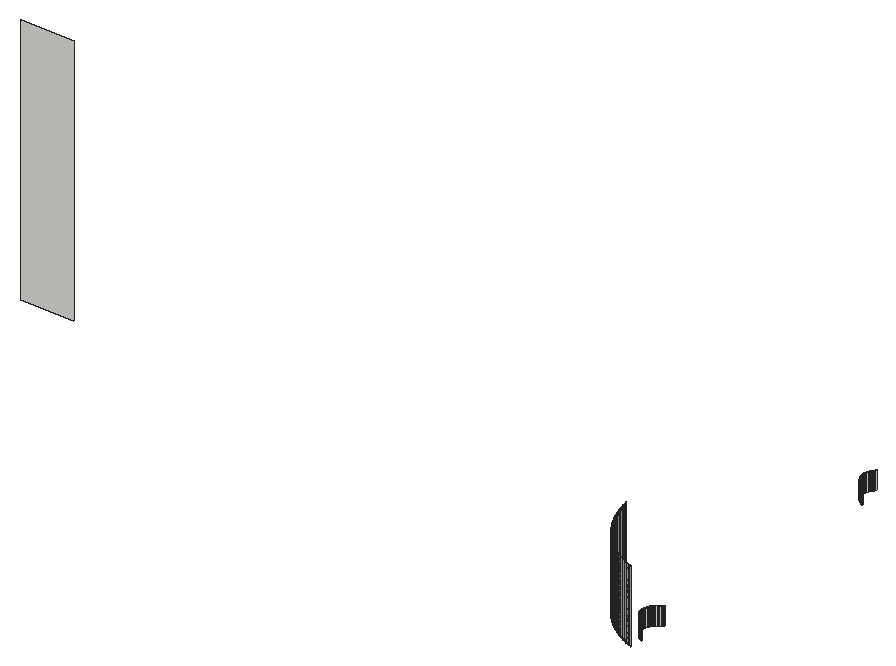
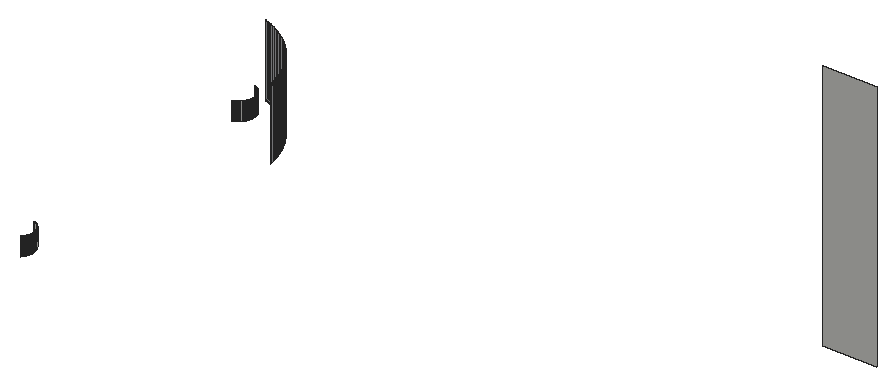
# SketchUp Ruby script. Lengths in inches.
U = 1.inch
M = Sketchup.active_model
def pt(a) = Geom::Point3d.new(a.map { |v| v * U })
def face(e, loops, mat)
  f = e.add_face(loops[0].map { |a| pt(a) })
  loops[1..].each { |l| e.add_face(l.map { |a| pt(a) }).erase! }
  f.material = f.back_material = mat if mat
  f
end
# faces: each face lists its corners as indices into pts; further lists are holes
def faces(e, pts, list, mat = nil) = list.each { |f| face(e, (f[0].is_a?(Array) ? f : [f]).map { |l| l.map { |i| pts[i] } }, mat) }
# xy, xz, yz: faces in a plane at the given z, y or x. An outline is a flat list of corners, or four numbers for a rectangle; further outlines are holes
def ring(l) = l.size == 4 ? [[l[0], l[1]], [l[2], l[1]], [l[2], l[3]], [l[0], l[3]]] : l.each_slice(2).to_a
def flat(e, list, mat, &to3) = list.each { |f| face(e, (f[0].is_a?(Array) ? f : [f]).map { |l| ring(l).map { |u, v| to3.(u, v) } }, mat) }
def xy(e, z, list, mat = nil) = flat(e, list, mat) { |x, y| [x, y, z] }
def xz(e, y, list, mat = nil) = flat(e, list, mat) { |x, z| [x, y, z] }
def yz(e, x, list, mat = nil) = flat(e, list, mat) { |y, z| [x, y, z] }
def lines(e, pts, list) = list.each { |a, b| e.add_line(pt(pts[a]), pt(pts[b])) }
# prism: a flat outline (further loops are holes) pulled along v
def prism(e, loops, v, mat = nil)
  f = face(e, loops, mat); d = Geom::Vector3d.new(v.map { |x| x * U })
  f.pushpull(f.normal.samedirection?(d) ? d.length : -d.length)
end
def box(e, o, s, mat = nil) = prism(e, [[o, [o[0] + s[0], o[1], o[2]], [o[0] + s[0], o[1] + s[1], o[2]], [o[0], o[1] + s[1], o[2]]]], [0, 0, s[2]], mat)
def at(x, y, z, deg = 0) = Geom::Transformation.translation(pt([x, y, z])) * Geom::Transformation.rotation(ORIGIN, Z_AXIS, deg.degrees)
def axes(o, x, y, z) = Geom::Transformation.new([*x, 0, *y, 0, *z, 0, *pt(o).to_a, 1])
def part(name) = M.definitions.add(name)
# library, detail: a bought-in or finely detailed component or shape, given as its bounding box
def library(name, o, s) = part(name).tap { |d| box(d.entities, o, s) }
def detail(e, o, s) = box(e.add_group.entities, o, s)
def put(e, d, t, mat = nil) = e.add_instance(d, t).tap { |i| i.material = mat if mat }
def group(e, t, mat = nil) = e.add_group.tap { |g| g.transformation = t; g.material = mat if mat }.entities
root = M.entities
M.materials.add("1427 AP 686 ARMOUR-N").color = [184, 186, 189]
xz(root,135.92,[[9,372,18,414]])
yz(root,120.75,[[126.34,366,126.42,369],[126.42,366,126.5,369],[126.5,366,126.58,369],[126.58,366,126.66,369],[172.59,366,172.67,369],
  [172.67,366,172.75,369],[172.75,366,172.83,369],[172.83,366,172.91,369]])
p = [[122.33,121.98,366],[122.54,121.9,366],[122.54,121.9,378],[122.33,121.98,378],[122.12,122.05,366],[122.12,122.05,378],
  [121.7,122.21,366],[121.91,122.13,366],[121.91,122.13,378],[121.7,122.21,378],[121.49,122.29,366],[121.49,122.29,378],
  [121.29,122.38,366],[121.29,122.38,378],[121.09,122.47,366],[121.09,122.47,378],[120.88,122.5625,366],[120.88,122.5625,378],
  [120.68,122.66,366],[120.68,122.66,378],[120.48,122.75,366],[120.48,122.75,378],[120.28,122.85,366],[120.28,122.85,378],
  [120.08,122.96,366],[120.08,122.96,378],[119.89,123.06,366],[119.89,123.06,378],[119.69,123.17,366],[119.69,123.17,378],
  [119.5,123.28,366],[119.5,123.28,378],[119.31,123.39,366],[119.31,123.39,378],[119.12,123.51,366],[119.12,123.51,378],
  [118.93,123.62,366],[118.93,123.62,378],[118.74,123.74,366],[118.74,123.74,378],[118.56,123.87,366],[118.56,123.87,378],
  [118.37,123.99,366],[118.37,123.99,378],[118.1875,124.12,366],[118.1875,124.12,378],[118.01,124.25,366],[118.01,124.25,378],
  [122.4,124.15,366],[122.33,124.18,366],[122.33,124.18,369],[122.4,124.15,369],[122.48,124.12,366],[122.48,124.12,369],
  [122.55,124.1,366],[122.55,124.1,369],[122.63,124.08,366],[122.63,124.08,369],[117.83,124.38,366],[117.83,124.38,378],
  [122.1875,124.24,366],[122.12,124.27,366],[122.12,124.27,369],[122.1875,124.24,369],[122.26,124.21,366],[122.26,124.21,369],
  [121.98,124.35,366],[121.91,124.39,366],[121.91,124.39,369],[121.98,124.35,369],[122.05,124.31,366],[122.05,124.31,369],
  [117.65,124.51,366],[117.65,124.51,378],[121.84,124.43,366],[121.78,124.48,366],[121.78,124.48,369],[121.84,124.43,369],
  [117.48,124.65,366],[117.48,124.65,378],[121.72,124.52,366],[121.66,124.57,366],[121.66,124.57,369],[121.72,124.52,369],
  [117.3,124.79,366],[117.3,124.79,378],[121.6,124.625,366],[121.54,124.68,366],[121.54,124.68,369],[121.6,124.625,369],
  [121.48,124.73,366],[121.43,124.79,366],[121.43,124.79,369],[121.48,124.73,369],[117.13,124.93,366],[117.13,124.93,378],
  [121.375,124.85,366],[121.32,124.91,366],[121.32,124.91,369],[121.375,124.85,369],[116.96,125.07,366],[116.96,125.07,378],
  [121.27,124.97,366],[121.27,124.97,369],[121.23,125.03,366],[121.18,125.09,366],[121.18,125.09,369],[121.23,125.03,369],
  [116.79,125.22,366],[116.79,125.22,378],[121.14,125.16,366],[121.14,125.16,369],[116.625,125.37,366],[116.625,125.37,378],
  [121.1,125.23,366],[121.06,125.3,366],[121.06,125.3,369],[121.1,125.23,369],[121.02,125.37,366],[121.02,125.37,369],
  [116.46,125.52,366],[116.46,125.52,378],[120.99,125.4375,366],[120.96,125.51,366],[120.96,125.51,369],[120.99,125.4375,369],
  [116.3,125.67,366],[116.3,125.67,378],[120.93,125.58,366],[120.93,125.58,369],[120.9,125.65,366],[120.9,125.65,369],
  [116.14,125.82,366],[116.14,125.82,378],[120.87,125.73,366],[120.85,125.8,366],[120.85,125.8,369],[120.87,125.73,369],
  [115.98,125.98,366],[115.98,125.98,378],[120.83,125.88,366],[120.83,125.88,369],[120.81,125.95,366],[120.81,125.95,369],
  [115.82,126.14,366],[115.82,126.14,378],[120.79,126.03,366],[120.78,126.11,366],[120.78,126.11,369],[120.79,126.03,369],
  [115.67,126.3,366],[115.67,126.3,378],[120.77,126.1875,366],[120.77,126.1875,369],[120.76,126.26,366],[120.76,126.26,369],
  [115.52,126.46,366],[115.52,126.46,378],[120.75,126.34,366],[120.75,126.34,369],[115.37,126.625,366],[115.37,126.625,378],
  [115.22,126.79,366],[115.22,126.79,378],[120.75,126.66,366],[120.76,126.74,366],[120.76,126.74,369],[120.75,126.66,369],
  [120.77,126.8125,366],[120.77,126.8125,369],[115.07,126.96,366],[115.07,126.96,378],[120.78,126.89,366],[120.78,126.89,369],
  [120.79,126.97,366],[120.79,126.97,369],[114.93,127.13,366],[114.93,127.13,378],[120.81,127.05,366],[120.81,127.05,369],
  [120.83,127.12,366],[120.83,127.12,369],[114.79,127.3,366],[114.79,127.3,378],[120.85,127.2,366],[120.85,127.2,369],
  [120.87,127.27,366],[120.87,127.27,369],[114.65,127.48,366],[114.65,127.48,378],[120.9,127.35,366],[120.9,127.35,369],
  [120.93,127.42,366],[120.93,127.42,369],[120.96,127.49,366],[120.96,127.49,369],[114.51,127.65,366],[114.51,127.65,378],
  [120.99,127.5625,366],[120.99,127.5625,369],[121.02,127.63,366],[121.02,127.63,369],[121.06,127.7,366],[121.06,127.7,369],
  [114.38,127.83,366],[114.38,127.83,378],[121.1,127.77,366],[121.1,127.77,369],[114.25,128.01,366],[114.25,128.01,378],
  [121.14,127.84,366],[121.14,127.84,369],[121.18,127.91,366],[121.18,127.91,369],[121.23,127.97,366],[121.23,127.97,369],
  [114.12,128.1875,366],[114.12,128.1875,378],[121.27,128.03,366],[121.27,128.03,369],[121.32,128.09,366],[121.32,128.09,369],
  [121.375,128.15,366],[121.375,128.15,369],[113.99,128.37,366],[113.99,128.37,378],[121.43,128.21,366],[121.43,128.21,369],
  [121.48,128.27,366],[121.48,128.27,369],[121.54,128.32,366],[121.54,128.32,369],[121.6,128.375,366],[121.6,128.375,369],
  [113.87,128.56,366],[113.87,128.56,378],[121.66,128.43,366],[121.66,128.43,369],[121.72,128.48,366],[121.72,128.48,369],
  [121.78,128.52,366],[121.78,128.52,369],[121.84,128.57,366],[121.84,128.57,369],[113.74,128.74,366],[113.74,128.74,378],
  [121.91,128.61,366],[121.91,128.61,369],[121.98,128.65,366],[121.98,128.65,369],[113.62,128.93,366],[113.62,128.93,378],
  [122.05,128.69,366],[122.05,128.69,369],[122.12,128.73,366],[122.12,128.73,369],[122.1875,128.76,366],[122.1875,128.76,369],
  [122.26,128.79,366],[122.26,128.79,369],[122.33,128.82,366],[122.33,128.82,369],[122.4,128.85,366],[122.4,128.85,369],
  [113.51,129.12,366],[113.51,129.12,378],[122.48,128.88,366],[122.48,128.88,369],[122.55,128.9,366],[122.55,128.9,369],
  [113.39,129.31,366],[113.39,129.31,378],[113.28,129.5,366],[113.28,129.5,378],[113.17,129.69,366],[113.17,129.69,378],
  [113.06,129.89,366],[113.06,129.89,378],[112.96,130.08,366],[112.96,130.08,378],[112.85,130.28,366],[112.85,130.28,378],
  [112.75,130.48,366],[112.75,130.48,378],[112.66,130.68,366],[112.66,130.68,378],[112.5625,130.88,366],[112.5625,130.88,378],
  [112.47,131.09,366],[112.47,131.09,378],[112.38,131.29,366],[112.38,131.29,378],[112.29,131.49,366],[112.29,131.49,378],
  [112.21,131.7,366],[112.21,131.7,378],[112.13,131.91,366],[112.13,131.91,378],[112.05,132.12,366],[112.05,132.12,378],
  [111.98,132.33,366],[111.98,132.33,378],[111.9,132.54,366],[111.9,132.54,378],[111.83,132.75,366],[111.83,132.75,378],
  [111.76,132.96,366],[111.76,132.96,378],[111.7,133.17,366],[111.7,133.17,378],[111.64,133.39,366],[111.64,133.39,378],
  [111.58,133.6,366],[111.58,133.6,378],[111.52,133.82,366],[111.52,133.82,378],[111.47,134.03,366],[111.47,134.03,378],
  [111.42,134.25,366],[111.42,134.25,378],[111.37,134.47,366],[111.37,134.47,378],[111.33,134.68,366],[111.33,134.68,378],
  [111.28,134.9,366],[111.28,134.9,378],[122.55,170.35,366],[122.48,170.37,366],[122.48,170.37,369],[122.55,170.35,369],
  [122.33,170.43,366],[122.26,170.46,366],[122.26,170.46,369],[122.33,170.43,369],[122.4,170.4,366],[122.4,170.4,369],
  [122.12,170.52,366],[122.05,170.56,366],[122.05,170.56,369],[122.12,170.52,369],[122.1875,170.49,366],[122.1875,170.49,369],
  [121.91,170.64,366],[121.84,170.68,366],[121.84,170.68,369],[121.91,170.64,369],[121.98,170.6,366],[121.98,170.6,369],
  [121.78,170.73,366],[121.72,170.77,366],[121.72,170.77,369],[121.78,170.73,369],[121.66,170.82,366],[121.6,170.875,366],
  [121.6,170.875,369],[121.66,170.82,369],[121.54,170.93,366],[121.48,170.98,366],[121.48,170.98,369],[121.54,170.93,369],
  [121.43,171.04,366],[121.375,171.1,366],[121.375,171.1,369],[121.43,171.04,369],[121.32,171.16,366],[121.32,171.16,369],
  [121.27,171.22,366],[121.23,171.28,366],[121.23,171.28,369],[121.27,171.22,369],[121.18,171.34,366],[121.14,171.41,366],
  [121.14,171.41,369],[121.18,171.34,369],[121.1,171.48,366],[121.1,171.48,369],[121.06,171.55,366],[121.02,171.62,366],
  [121.02,171.62,369],[121.06,171.55,369],[120.99,171.6875,366],[120.99,171.6875,369],[120.96,171.76,366],[120.96,171.76,369],
  [120.93,171.83,366],[120.9,171.9,366],[120.9,171.9,369],[120.93,171.83,369],[120.87,171.98,366],[120.87,171.98,369],
  [120.85,172.05,366],[120.85,172.05,369],[120.83,172.13,366],[120.81,172.2,366],[120.81,172.2,369],[120.83,172.13,369],
  [120.79,172.28,366],[120.79,172.28,369],[120.78,172.36,366],[120.78,172.36,369],[120.77,172.4375,366],[120.76,172.51,366],
  [120.76,172.51,369],[120.77,172.4375,369],[120.75,172.59,366],[120.75,172.59,369],[120.75,172.91,366],[120.76,172.99,366],
  [120.76,172.99,369],[120.75,172.91,369],[120.77,173.0625,366],[120.77,173.0625,369],[120.78,173.14,366],[120.78,173.14,369],
  [120.79,173.22,366],[120.79,173.22,369],[120.81,173.3,366],[120.81,173.3,369],[120.83,173.37,366],[120.83,173.37,369],
  [120.85,173.45,366],[120.85,173.45,369],[120.87,173.52,366],[120.87,173.52,369],[120.9,173.6,366],[120.9,173.6,369],
  [120.93,173.67,366],[120.93,173.67,369],[120.96,173.74,366],[120.96,173.74,369],[120.99,173.8125,366],[120.99,173.8125,369],
  [121.02,173.88,366],[121.02,173.88,369],[121.06,173.95,366],[121.06,173.95,369],[121.1,174.02,366],[121.1,174.02,369],
  [121.14,174.09,366],[121.14,174.09,369],[121.18,174.16,366],[121.18,174.16,369],[121.23,174.22,366],[121.23,174.22,369],
  [121.27,174.28,366],[121.27,174.28,369],[121.32,174.34,366],[121.32,174.34,369],[121.375,174.4,366],[121.375,174.4,369],
  [121.43,174.46,366],[121.43,174.46,369],[121.48,174.52,366],[121.48,174.52,369]]
faces(root,p,[[0,1,2,3],[4,0,3,5],[6,7,8,9],[7,4,5,8],[10,6,9,11],[12,10,11,13],[14,12,13,15],[16,14,15,17],
  [18,16,17,19],[20,18,19,21],[22,20,21,23],[24,22,23,25],[26,24,25,27],[28,26,27,29],[30,28,29,31],[32,30,31,33],
  [34,32,33,35],[36,34,35,37],[38,36,37,39],[40,38,39,41],[42,40,41,43],[44,42,43,45],[46,44,45,47],[58,46,47,59],
  [72,58,59,73],[78,72,73,79],[84,78,79,85],[94,84,85,95],[100,94,95,101],[108,100,101,109],[112,108,109,113],[120,112,113,121],
  [126,120,121,127],[132,126,127,133],[138,132,133,139],[144,138,139,145],[150,144,145,151],[156,150,151,157],[160,156,157,161],[162,160,161,163],
  [170,162,163,171],[176,170,171,177],[182,176,177,183],[188,182,183,189],[196,188,189,197],[204,196,197,205],[208,204,205,209],[216,208,209,217],
  [224,216,217,225],[234,224,225,235],[244,234,235,245],[250,244,245,251],[264,250,251,265],[270,264,265,271],[272,270,271,273],[274,272,273,275],
  [276,274,275,277],[278,276,277,279],[280,278,279,281],[282,280,281,283],[284,282,283,285],[286,284,285,287],[288,286,287,289],[290,288,289,291],
  [292,290,291,293],[294,292,293,295],[296,294,295,297],[298,296,297,299],[300,298,299,301],[302,300,301,303],[304,302,303,305],[306,304,305,307],
  [308,306,307,309],[310,308,309,311],[312,310,311,313],[314,312,313,315],[316,314,315,317],[318,316,317,319],[320,318,319,321],[322,320,321,323],
  [324,322,323,325]],"1427 AP 686 ARMOUR-N")
faces(root,p,[[48,49,50,51],[52,48,51,53],[54,52,53,55],[56,54,55,57],[60,61,62,63],[64,60,63,65],[49,64,65,50],[66,67,68,69],
  [70,66,69,71],[61,70,71,62],[74,75,76,77],[67,74,77,68],[80,81,82,83],[75,80,83,76],[86,87,88,89],[81,86,89,82],
  [90,91,92,93],[87,90,93,88],[96,97,98,99],[91,96,99,92],[97,102,103,98],[104,105,106,107],[102,104,107,103],[105,110,111,106],
  [114,115,116,117],[110,114,117,111],[115,118,119,116],[122,123,124,125],[118,122,125,119],[123,128,129,124],[128,130,131,129],[134,135,136,137],
  [130,134,137,131],[135,140,141,136],[140,142,143,141],[146,147,148,149],[142,146,149,143],[147,152,153,148],[152,154,155,153],[154,158,159,155],
  [164,165,166,167],[165,168,169,166],[168,172,173,169],[172,174,175,173],[174,178,179,175],[178,180,181,179],[180,184,185,181],[184,186,187,185],
  [186,190,191,187],[190,192,193,191],[192,194,195,193],[194,198,199,195],[198,200,201,199],[200,202,203,201],[202,206,207,203],[206,210,211,207],
  [210,212,213,211],[212,214,215,213],[214,218,219,215],[218,220,221,219],[220,222,223,221],[222,226,227,223],[226,228,229,227],[228,230,231,229],
  [230,232,233,231],[232,236,237,233],[236,238,239,237],[238,240,241,239],[240,242,243,241],[242,246,247,243],[246,248,249,247],[248,252,253,249],
  [252,254,255,253],[254,256,257,255],[256,258,259,257],[258,260,261,259],[260,262,263,261],[262,266,267,263],[266,268,269,267],[326,327,328,329],
  [330,331,332,333],[334,330,333,335],[327,334,335,328],[336,337,338,339],[340,336,339,341],[331,340,341,332],[342,343,344,345],[346,342,345,347],
  [337,346,347,338],[348,349,350,351],[343,348,351,344],[352,353,354,355],[349,352,355,350],[356,357,358,359],[353,356,359,354],[360,361,362,363],
  [357,360,363,358],[361,364,365,362],[366,367,368,369],[364,366,369,365],[370,371,372,373],[367,370,373,368],[371,374,375,372],[376,377,378,379],
  [374,376,379,375],[377,380,381,378],[380,382,383,381],[384,385,386,387],[382,384,387,383],[385,388,389,386],[388,390,391,389],[392,393,394,395],
  [390,392,395,391],[393,396,397,394],[396,398,399,397],[400,401,402,403],[398,400,403,399],[401,404,405,402],[406,407,408,409],[407,410,411,408],
  [410,412,413,411],[412,414,415,413],[414,416,417,415],[416,418,419,417],[418,420,421,419],[420,422,423,421],[422,424,425,423],[424,426,427,425],
  [426,428,429,427],[428,430,431,429],[430,432,433,431],[432,434,435,433],[434,436,437,435],[436,438,439,437],[438,440,441,439],[440,442,443,441],
  [442,444,445,443],[444,446,447,445],[446,448,449,447],[448,450,451,449],[450,452,453,451]])
